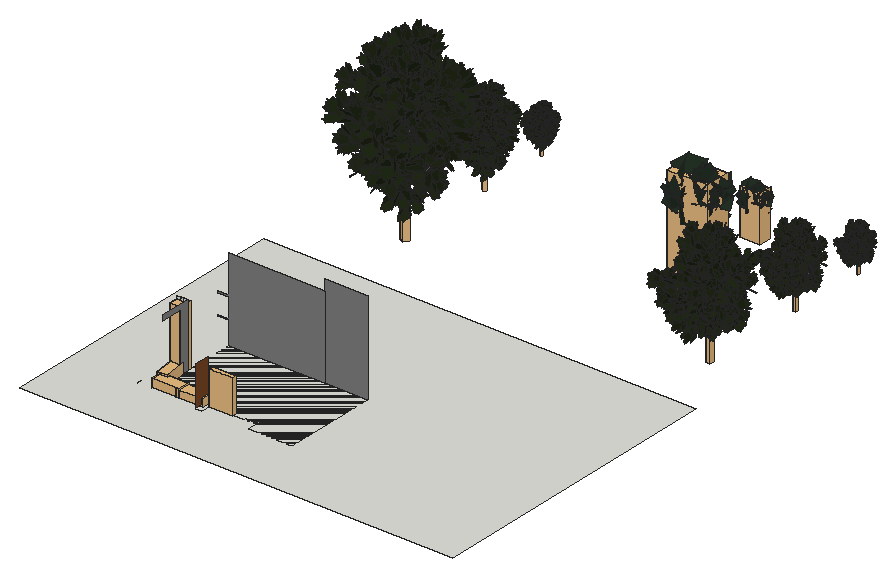
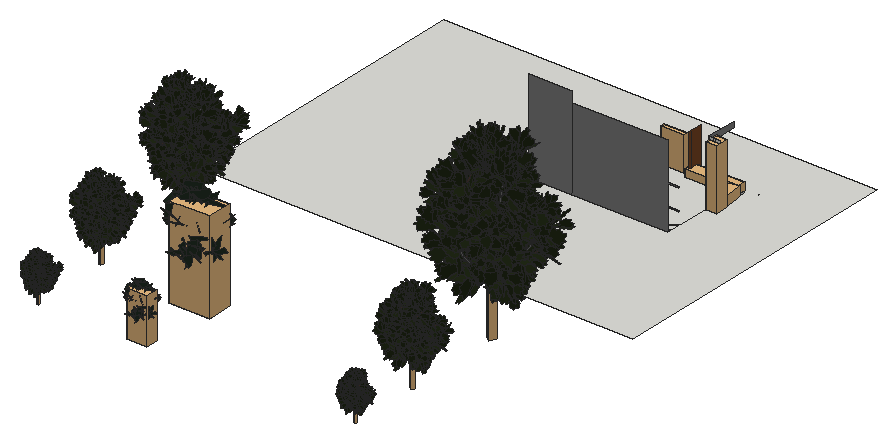
# SketchUp Ruby script. Lengths in inches.
U = 1.inch
M = Sketchup.active_model
def pt(a) = Geom::Point3d.new(a.map { |v| v * U })
def face(e, loops, mat)
  f = e.add_face(loops[0].map { |a| pt(a) })
  loops[1..].each { |l| e.add_face(l.map { |a| pt(a) }).erase! }
  f.material = f.back_material = mat if mat
  f
end
# faces: each face lists its corners as indices into pts; further lists are holes
def faces(e, pts, list, mat = nil) = list.each { |f| face(e, (f[0].is_a?(Array) ? f : [f]).map { |l| l.map { |i| pts[i] } }, mat) }
# xy, xz, yz: faces in a plane at the given z, y or x. An outline is a flat list of corners, or four numbers for a rectangle; further outlines are holes
def ring(l) = l.size == 4 ? [[l[0], l[1]], [l[2], l[1]], [l[2], l[3]], [l[0], l[3]]] : l.each_slice(2).to_a
def flat(e, list, mat, &to3) = list.each { |f| face(e, (f[0].is_a?(Array) ? f : [f]).map { |l| ring(l).map { |u, v| to3.(u, v) } }, mat) }
def xy(e, z, list, mat = nil) = flat(e, list, mat) { |x, y| [x, y, z] }
def xz(e, y, list, mat = nil) = flat(e, list, mat) { |x, z| [x, y, z] }
def yz(e, x, list, mat = nil) = flat(e, list, mat) { |y, z| [x, y, z] }
def lines(e, pts, list) = list.each { |a, b| e.add_line(pt(pts[a]), pt(pts[b])) }
# prism: a flat outline (further loops are holes) pulled along v
def prism(e, loops, v, mat = nil)
  f = face(e, loops, mat); d = Geom::Vector3d.new(v.map { |x| x * U })
  f.pushpull(f.normal.samedirection?(d) ? d.length : -d.length)
end
def box(e, o, s, mat = nil) = prism(e, [[o, [o[0] + s[0], o[1], o[2]], [o[0] + s[0], o[1] + s[1], o[2]], [o[0], o[1] + s[1], o[2]]]], [0, 0, s[2]], mat)
def at(x, y, z, deg = 0) = Geom::Transformation.translation(pt([x, y, z])) * Geom::Transformation.rotation(ORIGIN, Z_AXIS, deg.degrees)
def axes(o, x, y, z) = Geom::Transformation.new([*x, 0, *y, 0, *z, 0, *pt(o).to_a, 1])
def part(name) = M.definitions.add(name)
# library, detail: a bought-in or finely detailed component or shape, given as its bounding box
def library(name, o, s) = part(name).tap { |d| box(d.entities, o, s) }
def detail(e, o, s) = box(e.add_group.entities, o, s)
def put(e, d, t, mat = nil) = e.add_instance(d, t).tap { |i| i.material = mat if mat }
def group(e, t, mat = nil) = e.add_group.tap { |g| g.transformation = t; g.material = mat if mat }.entities
root = M.entities
M.materials.add("Color_D09").color = [86, 59, 49]
M.materials.add("Door").color = [117, 63, 33]
M.materials.add("Green ash – green texture").color = [33, 41, 22]
M.materials.add("[0133_Gray]").color = [128, 128, 128]
M.materials.add("[Color_005]1").color = [114, 114, 114]
M.materials.add("[Grass Dark Green]").color = [106, 157, 55]
M.materials.add("[Wood Veneer 01]").color = [120, 70, 37]
M.materials.add("euc leaf02").color = [35, 48, 36]
c1 = part("Component\#32")
xz(c1.entities,0,[[2.54,0,9.87,0.64,10.99,2.07,11.4,3.42,15.13,2.28,14.48,4.31,16.14,5.21,16.14,6.08,19.81,7.28,19.6,9.67,17.45,11.49,17.45,12.16,18.82,14.37,17.48,14.37,14.41,13.66,14.41,15.23,12.5625,17.49,9.84,15.21,8.9,13.85,7.74,13.625,7.35,12.68,6.87,13.02,6.35,12.27,5.92,10.47,4.2,7.42,2.84,6.89,0,2.38,0.07,1.59,2.8125,4.94,3.37,3.59,2.54,3.37,2.12,2.22]],"Green ash – green texture")
c2 = part("Component\#31")
xz(c2.entities,0,[[1.1,0,1.61,0,2.73,1.11,4.34,2.72,5.21,6.36,5.85,7.16,6.35,6.9375,6.85,8.05,8.03,8.05,8.625,9.25,10.11,11.7,9.56,13.83,9.56,15.84,7.83,15.84,6.03,14.37,5.31,16.54,4.4375,17.39,1.45,14.31,0,9.15,1.4,5.18,3.01,6.08,1.98,1.39]],"Green ash – green texture")
c3 = part("Component\#30")
put(c3.entities,c1,axes([0,7.77,0],[1,0,0],[0,0.89571,0.44464],[0,-0.44464,0.89571]))
put(c3.entities,c2,axes([2.15,6.37,5.26],[0.57629,-0.80824,0.12095],[0.79263,0.51673,-0.3236],[0.19905,0.28236,0.93843]))
c4 = part("Component\#33")
put(c4.entities,c3,axes([-4.97,-3.22,4.05],[0.69883,-0.69034,0.18725],[0.53248,0.3273,-0.7806],[0.47759,0.64522,0.59632]))
c5 = part("Component\#35")
put(c5.entities,c4,axes([0,5.2,2.2],[1,0,0],[0,0.90259,0.43051],[0,-0.43051,0.90259]))
c6 = part("leaf group 2")
put(c6.entities,c5,axes([-11.99,4.41,-4.35],[2.22014,-0.82385,1.14017],[1.36501,1.77637,-1.37441],[-0.33979,1.75315,1.92841]))
c7 = part("Component\#37")
put(c7.entities,c6,axes([-5.27,11.65,1.68],[-0.48323,0.10636,-0.43072],[-0.11515,-0.64511,-0.03012],[-0.42845,0.05342,0.49388]))
c8 = part("Component\#36")
xz(c8.entities,0,[[0.64,0,0,0.1875,4.21,2.81,8.59,4.11,12.8,4.11,19.57,2.81,12.8,3.73,8.59,3.73,4.21,2.3125]],"Color_D09")
c9 = part("Leafy twig")
put(c9.entities,c7,axes([23.53,12.57,24.85],[0.06536,-0.90475,-0.42089],[0.61791,-0.2945,0.72901],[-0.78353,-0.30772,0.53981]))
put(c9.entities,c7,axes([22.7,12.25,24.83],[-0.47146,-0.89493,0.11311],[0.80135,-0.48549,-0.35888],[0.36776,-0.0521,0.90651]))
put(c9.entities,c7,axes([24.25,0.65,20.83],[0.8253,-0.50372,0.24924],[0.23848,0.71461,0.65749],[-0.51157,-0.48438,0.71194]))
put(c9.entities,c7,axes([23.54,-2.45,18.63],[0.04689,-0.92492,0.3511],[0.72122,-0.28285,-0.64421],[0.71641,0.2674,0.65188]))
put(c9.entities,c7,axes([22.39,16.15,27.04],[-0.5311,-0.82173,0.2419],[0.41574,0.01583,0.89559],[-0.77461,0.50499,0.40813]))
put(c9.entities,c8,axes([22.76,-5.09,13.48],[0,1.66539,0.44624],[-1.72414,0,0],[0,-0.44624,1.66539]))
c10 = part("Bare twig")
p = [[0,0,0.13],[0.41,0.77,0],[4.07,2.79,10.125],[3.73,2.15,10.23],[7.66,4.77,23.875],[7.4,4.27,23.96],
  [8.6875,5.26,35.99],[8.5,4.91,36.05],[8.32,4.9375,46.95],[8.21,4.74,46.98]]
faces(c10.entities,p,[[0,1,2,3],[3,2,4,5],[4,6,7,5],[6,8,9,7]],"[Color_005]1")
c11 = part("Leafy twig \#1")
put(c11.entities,c10,axes([3.13,0.17,-0.45],[3.38032,6.88592,0.52481],[-5.85488,3.97559,0.303],[0,-1.35912,3.54524]))
put(c11.entities,c7,axes([0.37,31.375,148.94],[0.47772,0.64064,-1.51139],[2.85768,-0.62659,0.20284],[-0.43926,-3.3797,-0.3241]))
c12 = part("Ash branch")
put(c12.entities,c9,axes([28.11,72.66,46.26],[0.77413,-0.41274,-0.47998],[0.6311,0.56229,0.53435],[0.04934,-0.71657,0.69577]))
put(c12.entities,c9,axes([31.25,3.94,9.17],[0.73236,0.67893,0.05208],[-0.46223,0.55185,-0.69413],[-0.5,0.48428,0.71797]))
put(c12.entities,c9,axes([20.16,84.84,57.95],[0.96628,0.19619,0.16678],[-0.2575,0.73909,0.62245],[-0.00115,-0.6444,0.76469]))
put(c12.entities,c9,axes([30.13,29.18,11.93],[0.86603,0.2796,0.41452],[0,0.82904,-0.55919],[-0.5,0.48428,0.71797]))
put(c12.entities,c9,axes([47.67,28.63,-3.7],[0.1205,-0.71255,0.69119],[0.96646,0.24327,0.08231],[-0.2268,0.65809,0.71797]))
put(c12.entities,c9,axes([48.76,50.64,76.31],[-0.6716,0.46861,-0.57389],[0.01402,0.78248,0.62252],[0.74078,0.41004,-0.53209]))
put(c12.entities,c11,axes([42.34,0,10.34],[0.39368,0,0],[0,0.22544,-0.24092],[0,0.54032,0.50562]))
put(c12.entities,c9,axes([64.51,80.82,101.08],[-0.99604,0.06562,-0.06004],[-0.0106,0.58266,0.81265],[0.08831,0.81006,-0.57966]))
c13 = part("Ash branch \#2")
put(c13.entities,c9,axes([-3.64,36.17,23.18],[0.95801,0.10249,0.26779],[-0.28581,0.41631,0.86313],[-0.02302,-0.90343,0.42812]))
put(c13.entities,c9,axes([13.16,55.79,39.92],[0.70711,-0.61725,0.34497],[0,0.48786,0.87292],[-0.70711,-0.61725,0.34497]))
put(c13.entities,c11,axes([18.8125,5.17,0.46],[0.25503,0,0],[0,0.20007,-0.0752],[0,0.16866,0.44872]))
put(c13.entities,c9,axes([23.62,-10.17,21.5],[-0.56253,0.81775,0.12181],[0.38738,0.13053,0.91263],[0.73041,0.56057,-0.39021]))
put(c13.entities,c9,axes([45.18,27.18,68.96],[-0.96593,-0.22593,0.12627],[0.12295,0.02876,0.992],[-0.22775,0.97372,0]))
c14 = library("Tree trunk",[-6.35,9.4375,-76.57],[12.56,13.68,315.77])
c15 = part("Ash branch \#3")
put(c15.entities,c11,axes([21.47,3.93,0.22],[0.25503,0,0],[0,0.21068,-0.03601],[0,0.08077,0.47252]))
put(c15.entities,c9,axes([-4.05,13.6875,55.34],[0.70711,0.70373,-0.069],[0,0.09758,0.99523],[0.70711,-0.70373,0.069]))
put(c15.entities,c9,axes([6.52,33.54,18.07],[0.92587,-0.37604,0.03687],[0,0.09758,0.99523],[-0.37784,-0.92145,0.09035]))
c16 = part("Ash branch \#1")
put(c16.entities,c9,axes([26.17,74.02,40.56],[0.25882,-0.64004,0.72344],[0,0.74896,0.66262],[-0.96593,-0.1715,0.19384]))
put(c16.entities,c9,axes([6.38,24.03,55.81],[-0.04786,0.8645,-0.50035],[0.15558,0.50126,0.85119],[0.98666,-0.03711,-0.15849]))
put(c16.entities,c11,axes([17.68,0,1.01],[0.32282,0,0],[0,0.21407,-0.16545],[0,0.37107,0.48011]))
put(c16.entities,c9,axes([-9.1875,31.15,28.07],[0.82314,0.37626,-0.42529],[0,0.74896,0.66262],[0.56784,-0.54543,0.61649]))
put(c16.entities,c9,axes([0.54,-12.07,9.94],[0.19622,0.90478,-0.37799],[-0.67396,0.40444,0.61823],[0.71224,0.13344,0.68914]))
put(c16.entities,c9,axes([7.34,9.15,39.57],[0.05153,0.73872,-0.67204],[0.38679,0.60565,0.6954],[0.92072,-0.29578,-0.25452]))
put(c16.entities,c9,axes([36.2,51.23,15.73],[-0.18626,-0.35374,0.91661],[-0.31641,0.90483,0.2849],[-0.93016,-0.23696,-0.28046]))
c17 = part("Tree")
put(c17.entities,c12,axes([209.16,146.26,190.79],[-0.28773,1.46382,-0.87256],[-1.6259,0,0.48096],[0.49836,0.84514,1.51132]))
put(c17.entities,c12,axes([134.38,215.25,141.01],[1.59145,0,0],[0,1.58386,0.23671],[0,-0.32836,1.69393]))
put(c17.entities,c13,axes([178.04,237.71,388.46],[0,-1.63474,0],[1.63474,0,0],[0,0,1.78187]))
put(c17.entities,c12,axes([256.65,171.18,211.31],[-1.36815,1.04036,0],[-1.04036,-1.36815,0],[0,0,1.87346]))
put(c17.entities,c12,axes([167.11,160.33,284.63],[0.63716,1.20925,-0.47341],[-1.25908,0.71729,0.13762],[0.43501,0.34501,1.46674]))
put(c17.entities,c14,axes([199.97,188.06,127.43],[1.59145,0,0],[0,1.59145,0],[0,0,1.66425]))
put(c17.entities,c12,axes([275.77,218.4,281.93],[-1.57517,-0.28132,-0.44593],[0.06295,-1.50318,0.62621],[-0.42383,0.67416,1.53786]))
put(c17.entities,c12,axes([190.14,288,146.64],[0.35111,-1.78964,0],[1.72866,0.33915,0.47202],[-0.50488,-0.09905,1.92016]))
put(c17.entities,c12,axes([257.54,236.65,165.53],[-1.29152,-0.54158,0],[0.54158,-1.29152,0],[0,0,1.52652]))
put(c17.entities,c12,axes([175.36,274.13,265.04],[0.47642,-1.31213,-0.12271],[1.30597,0.45529,0.24003],[-0.16973,-0.17989,1.50253]))
put(c17.entities,c13,axes([228.65,212.14,385.35],[-1.53723,0.39369,-0.12111],[-0.39786,-1.55122,0.00748],[-0.10661,0.11241,1.71849]))
put(c17.entities,c15,axes([179.375,247.82,455.73],[0.79573,-1.37824,0],[1.37824,0.79573,0],[0,0,1.73468]))
put(c17.entities,c15,axes([220.2,190.4,436.52],[-0.90108,1.29724,0.19482],[-1.26794,-0.9219,0.27414],[0.36658,0,1.69551]))
put(c17.entities,c16,axes([195.4,185.625,330.61],[0,1.80471,0],[-1.731,0,0.5105],[0.55644,0,1.88679]))
put(c17.entities,c16,axes([180.07,237.23,322.66],[1.03006,-1.73903,-0.39964],[1.71651,0.8636,0.79163],[-0.4607,-0.67055,2.05597]))
put(c17.entities,c12,axes([252.86,167.09,121.2],[-1.29065,1.04142,0.30989],[-1.03312,-1.28343,0.15838],[0.47872,-0.11505,1.68865]))
put(c17.entities,c12,axes([145.45,238.15,252.03],[1.32497,-0.45364,0],[0.45364,1.32497,0],[0,0,1.52652]))
put(c17.entities,c16,axes([222.54,228.83,294],[-1.20488,-1.04179,0.83261],[1.23186,-1.24114,0.27288],[0.38905,0.70343,1.7146]))
put(c17.entities,c16,axes([223.77,224.36,314.875],[-1.40575,-0.68986,-0.30962],[0.56266,-1.37824,0.6133],[-0.4899,0.39658,1.59284]))
put(c17.entities,c16,axes([166.75,216.1,346.53],[1.65511,0,0],[0,1.6365,0.2475],[0,-0.26977,1.78379]))
put(c17.entities,c13,axes([162.33,209.39,372.71],[1.56679,-0.27909,0],[0.27909,1.56679,0],[0,0,1.73468]))
put(c17.entities,c13,axes([203.35,171.86,386.35],[0.15996,1.63137,0],[-1.63137,0.15996,0],[0,0,1.78672]))
c18 = part("Green Ash")
put(c18.entities,c14,axes([99.99,94.03,63.71],[0.79573,0,0],[0,0.79573,0],[0,0,0.83213]))
put(c18.entities,c13,axes([101.67,85.93,193.17],[0.07998,0.81569,0],[-0.81569,0.07998,0],[0,0,0.89336]))
put(c18.entities,c13,axes([89.02,118.86,194.23],[0,-0.81737,0],[0.81737,0,0],[0,0,0.89093]))
put(c18.entities,c12,axes([137.88,109.2,140.96],[-0.78759,-0.14066,-0.22296],[0.03147,-0.75159,0.31311],[-0.21191,0.33708,0.76893]))
put(c18.entities,c12,axes([67.1875,107.625,70.5],[0.79573,0,0],[0,0.79193,0.11835],[0,-0.16418,0.84696]))
put(c18.entities,c12,axes([104.58,73.13,95.39],[-0.14386,0.73191,-0.43628],[-0.81295,0,0.24048],[0.24918,0.42257,0.75566]))
put(c18.entities,c12,axes([128.33,85.59,105.66],[-0.68407,0.52018,0],[-0.52018,-0.68407,0],[0,0,0.93673]))
put(c18.entities,c12,axes([128.77,118.32,82.77],[-0.64576,-0.27079,0],[0.27079,-0.64576,0],[0,0,0.76326]))
put(c18.entities,c13,axes([114.32,106.07,192.67],[-0.76861,0.19684,-0.06056],[-0.19893,-0.77561,0.00374],[-0.0533,0.05621,0.85925]))
put(c18.entities,c12,axes([83.56,80.16,142.32],[0.31858,0.60462,-0.23671],[-0.62954,0.35865,0.06881],[0.21751,0.1725,0.73337]))
put(c18.entities,c13,axes([81.16,104.7,186.36],[0.7834,-0.13954,0],[0.13954,0.7834,0],[0,0,0.86734]))
put(c18.entities,c16,axes([97.7,92.8125,165.31],[0,0.90235,0],[-0.8655,0,0.25525],[0.27822,0,0.94339]))
put(c18.entities,c12,axes([87.68,137.07,132.52],[0.23821,-0.65607,-0.06135],[0.65299,0.22764,0.12002],[-0.08486,-0.08995,0.75126]))
put(c18.entities,c15,axes([89.6875,123.91,227.86],[0.39786,-0.68912,0],[0.68912,0.39786,0],[0,0,0.86734]))
put(c18.entities,c12,axes([95.07,144,73.32],[0.17556,-0.89482,0],[0.86433,0.16957,0.23601],[-0.25244,-0.04953,0.96008]))
put(c18.entities,c15,axes([110.1,95.2,218.26],[-0.45054,0.64862,0.09741],[-0.63397,-0.46095,0.13707],[0.18329,0,0.84775]))
put(c18.entities,c16,axes([90.03,118.62,161.33],[0.51503,-0.86951,-0.19982],[0.85825,0.4318,0.39581],[-0.23035,-0.33528,1.02798]))
put(c18.entities,c16,axes([83.38,108.05,173.27],[0.82756,0,0],[0,0.81825,0.12375],[0,-0.13489,0.89189]))
put(c18.entities,c16,axes([111.27,114.42,147],[-0.60244,-0.5209,0.41631],[0.61593,-0.62057,0.13644],[0.19452,0.35171,0.8573]))
put(c18.entities,c12,axes([126.43,83.55,60.6],[-0.64533,0.52071,0.15494],[-0.51656,-0.64172,0.07919],[0.23936,-0.05752,0.84432]))
put(c18.entities,c16,axes([111.89,112.18,157.4375],[-0.70287,-0.34493,-0.15481],[0.28133,-0.68912,0.30665],[-0.24495,0.19829,0.79642]))
put(c18.entities,c12,axes([72.73,119.08,126.01],[0.66249,-0.22682,0],[0.22682,0.66249,0],[0,0,0.76326]))
c19 = library("Group8",[-183.25,9.15,0],[25.91,56.79,43.93])
c20 = library("Group13",[-203.48,36.63,0],[29.68,67.31,50.64])
c21 = part("House+plant_11")
xy(c21.entities,0,[[-51.0625,-134.25,1040.6875,632.93]])
put(c21.entities,c19,at(-20.85,102.1,-20.91,-173.7))
put(c21.entities,c20,at(112.35,-141.89,-30.93,-90))
put(c21.entities,c20,at(172.12,-141.81,-32.82,-90))
c22 = library("GoldenBamboo",[-21.19,-21.7,-0.46],[44.22,41.02,72.81])
c23 = library("Group\#3",[0,0,0],[259.75,161.77,589.29])
c24 = part("Blue Gum")
p = [[271.53,158.18,378.25],[270.5625,158.71,380.69],[270.37,158.83,381.17],[272.73,162.06,384.51],[213.85,150.08,152.75],[212.24,149.06,149.65],
  [150.49,110.24,344.32],[151.97,108.18,342.21],[217.47,152.58,206.91],[209.32,150.04,213.6],[153.27,112.37,338.72],[213.34,156.04,223.13],
  [212.17,155.27,219.89],[213.66,148.52,337.14],[212.6875,151.94,345.88],[201.33,160.36,0],[198.82,151.26,0.01],[228.58,150.59,468.55],
  [228.91,150.53,474.28],[226.95,148.99,472.86]]
faces(c24.entities,p,[[0,1,2],[1,0,3],[3,2,1]])
lines(c24.entities,p,[[4,5],[6,7],[8,9],[10,6],[7,10],[11,12],[13,14],[15,16],[17,18],[19,17],[18,19]])
put(c24.entities,c23,axes([324.42,234.92,0.08],[-1,0,-0.00067],[0,-1,0.00003],[-0.00067,0.00003,1]))
g1 = group(c24.entities,at(392.72,299.04,214.24))
p = [[-190.24,-45.24,49.75],[-155.8,-83.51,-0.1],[-171.1,-117.4,15.86],[-186.4,-151.3,31.82],[-220.85,-113.03,81.67],[-197.84,-62.08,57.68],
  [-156.97,-85.38,90],[-134.58,-101.98,23.98],[-207.62,-132.83,7.74],[-230.01,-116.24,73.77],[-175.11,-93.05,85.97],[-155.875,-47.35,89.82],
  [-171.875,-81.0625,28.63],[-175.09,-115.85,49.06],[-178.3125,-150.63,69.48],[-162.3125,-116.92,130.67],[-157.47,-64.63,99.96],[-108.86,-93.44,91.87],
  [-142.19,-103.1875,29.18],[-207.99,-128.51,68.93],[-174.66,-118.76,131.62],[-125.2,-99.73,101.74],[-105.25,-143.93,101.02],[-118.65,-122.91,33.83],
  [-139.46,-91.34,48.24],[-160.28,-59.76,62.65],[-146.87,-80.78,129.84],[-115.59,-128.24,108.18],[-69.65,-64.39,98.91],[-102.98,-74.13,36.22],
  [-135.88,-86.79,56.09],[-168.78,-99.45,75.97],[-135.45,-89.7,138.66],[-85.99,-70.68,108.78],[-206,0,112.1],[-205.51,-55.1,41.09],
  [-219.69,-93.37,71.26],[-233.87,-131.63,101.43],[-234.36,-76.53,172.4375],[-220.18,-38.26,142.27],[-213.05,-19.01,127.09],[-58.99,-92.56,99.73],
  [-109.77,-114.37,54.1],[-132.54,-82.69,64.86],[-155.3,-51.01,75.61],[-104.53,-29.2,121.24],[-70.31,-76.82,105.07],[-84.85,-14.67,104.44],
  [-93.72,-70.0625,59.84],[-130.5,-76.32,75.5],[-167.29,-82.57,91.16],[-158.42,-27.18,135.76],[-103.12,-17.78,112.22],[-170.99,-48.24,149.78],
  [-170.5,-103.34,78.77],[-268.88,-83.39,63.75],[-269.37,-28.29,134.76],[-195.43,-43.28,146.05],[-119.44,-162.62,158.17],[-165.08,-157.98,109.24],
  [-139.69,-139.86,87.75],[-114.31,-121.74,66.26],[-68.68,-126.38,115.19],[-94.0625,-144.5,136.68],[-106.83,-153.62,147.5],[-83.43,-178.22,123.11],
  [-129.0625,-173.58,74.18],[-150.32,-106.13,101.32],[-104.69,-110.78,150.25],[-88.71,-161.47,129.85],[-153.18,-33.52,154.23],[-187.55,-61.6,76.08],
  [-205.14,-103.18,99.27],[-222.72,-144.75,122.47],[-188.35,-116.67,200.62],[-170.77,-75.09,177.42],[-161.92,-54.17,165.75],[-126.95,-97.9375,165.85],
  [-161.32,-126.02,87.7],[-248.95,-80.33,110.85],[-214.58,-52.25,189],[-148.72,-86.59,171.6],[-365.27,-93.53,149.96],[-339.43,-156.16,87.91],
  [-290.4375,-139.67,92.34],[-241.45,-123.17,96.77],[-267.29,-60.54,158.83],[-340.93,-85.33,152.16],[-220,-209.94,88.83],[-192.18,-284.625,134.55],
  [-202.3,-275.33,156.35],[-232.93,-247.2,222.33],[-260.75,-172.52,176.61],[-240.375,-191.23,132.72],[-392.72,-100.24,198.19],[-366.88,-162.88,136.14],
  [-328.26,-131.57,121.3],[-289.64,-100.27,106.47],[-315.48,-37.63,168.52],[-373.54,-84.69,190.82],[-327.95,-161.62,221.67],[-317.1,-180.89,132.49],
  [-328.31,-131.57,120.9375],[-339.53,-82.25,109.39],[-350.38,-62.97,198.5625],[-333.52,-137.11,215.93],[-255.83,-236.76,152.47],[-329.61,-198.39,191.52],
  [-323.5,-175.58,181.2],[-305,-106.55,149.96],[-231.21,-144.93,110.9],[-243.52,-190.85,131.6875],[-205.5,-81.8,220.89],[-197.86,-85.86,131.43],
  [-243.5,-64.11,127],[-289.13,-42.35,122.57],[-296.77,-38.29,212.03],[-251.13,-60.04,216.46],[-228.17,-70.99,218.6875],[-234.33,-241.65,142.48],
  [-225.25,-222.09,231.79],[-228.94,-197.05,226.92],[-240.1,-121.29,212.17],[-249.18,-140.85,122.86],[-241.75,-191.25,132.67],[-227.68,-15.04,215.96],
  [-220.04,-19.1,126.5],[-266.95,-109.11,127.5],[-274.59,-105.04,216.95],[-239.33,-37.4,216.21],[-312.18,-35.14,201.88],[-307.82,-106.7,144.42],
  [-256.66,-99.36,139.9],[-205.5,-92.02,135.375],[-209.86,-20.46,192.83],[-286.77,-31.49,199.63],[-224.25,-107.3,143.78],[-158.47,-57.42,184.1],
  [-153.89,-76.52,200.79],[-140.05,-134.32,251.29],[-205.83,-184.2,210.96],[-215.04,-145.75,177.37],[-371.18,-63.42,218.95],[-318.87,-74.08,144.18],
  [-278.67,-86.3125,174.61],[-238.47,-98.55,205.04],[-290.78,-87.88,279.82],[-351.21,-69.49,234.07],[-314.82,-59.28,247.3],[-323.0625,-96.32,163.62],
  [-272.16,-89.61,156.15],[-221.26,-82.9,148.67],[-213.02,-45.87,232.35],[-289.54,-55.95,243.59],[-269.6,-260.65,169.64],[-261.02,-289.45,256.47],
  [-255.15,-265.53,264.0625],[-237.36,-193.15,287.04],[-245.94,-164.36,200.22],[-257.77,-212.5,184.93],[-219.98,-94.58,184.38],[-135.38,-92.14,220.14],
  [-132.93,-117.5625,216.66],[-125.5,-194.48,206.12],[-210.1,-196.92,170.36],[-242.72,-259.5,171.19],[-311.27,-292.91,222.44],[-317.8125,-269.04,229.65],
  [-337.62,-196.84,251.48],[-269.07,-163.43,200.23],[-255.89,-211.46,185.71],[-204.01,-188.2,177.79],[-188.33,-208.64,265.98],[-194.51,-184.59,272.89],
  [-213.23,-111.83,293.8125],[-228.92,-91.39,205.62],[-216.46,-139.79,191.7],[-111.12,-172.19,178.4],[-144.16,-223.61,247],[-146.96,-202.62,261.69],
  [-155.45,-139.1,306.14],[-122.41,-87.68,237.53],[-116.76,-129.9375,207.97],[-92.3,-219.25,321.53],[-140.07,-175.86,256.125],[-105.48,-191.84,220.91],
  [-70.89,-207.83,185.69],[-23.13,-251.22,251.1],[-75.12,-227.1875,304.03],[-95.32,-86.56,260.02],[-28.15,-67.53,258.27],[-24.95,-79.6,243.18],
  [-15.25,-116.11,197.51],[-82.42,-135.13,199.26],[-88.87,-110.84,229.64],[-230.35,-182.42,199.75],[-240.26,-200.67,289.25],[-235.09,-176.09,295.07],
  [-219.44,-101.74,312.67],[-209.53,-83.5,223.17],[-219.9375,-132.96,211.46],[-140.68,-151.65,266.01],[-78.24,-142.94,332.84],[-63.08,-129.17,317.2],
  [-17.2,-87.5,269.85],[-79.64,-96.22,203.02],[-110.16,-123.93,234.52],[-181.78,-155.46,254.29],[-197.87,-106.1875,330.15],[-215.8125,-92.48,317.72],
  [-270.1,-51.01,280.11],[-254.02,-100.28,204.25],[-217.9,-127.875,229.27],[-219.05,-237.83,228.68],[-246.19,-265.11,312.11],[-270.4375,-258.25,306.72],
  [-343.82,-237.49,290.4],[-316.68,-210.21,206.96],[-267.86,-224.02,217.82],[-221.64,-245.99,220.16],[-255.74,-296.14,289.1875],[-278.74,-284.87,286.3125],
  [-348.35,-250.78,277.61],[-314.25,-200.64,208.59],[-267.95,-223.32,214.37],[-214.08,-176.63,246.6],[-287.9,-162.75,299.5],[-289.8,-138.53,290.89],
  [-295.55,-65.24,264.85],[-221.72,-79.12,211.94],[-273.56,-277.41,225.52],[-332.72,-264.05,294.53],[-330.67,-238.52,291.65],[-324.47,-161.27,282.95],
  [-265.3,-174.62,213.93],[-269.43,-226.01,219.72],[-125.42,-280.5,273.74],[-154.49,-208.42,224.74],[-56.47,-175.26,217.08],[-27.39,-247.34,266.08],
  [-101.07,-272.26,271.84],[-137.08,-126.63,220.68],[-181.31,-63.4,270.55],[-159.07,-51.25,275.29],[-91.8,-14.51,289.63],[-47.57,-77.74,239.76],
  [-92.33,-102.1875,230.22],[-238.16,-243.49,222.62],[-218.34,-248.07,312.22],[-217.08,-222.36,313.49],[-213.28,-144.56,317.34],[-233.09,-139.97,227.74],
  [-235.625,-191.73,225.18],[-96.8,-128.7,236.99],[-25.62,-162.74,224.18],[-29.7,-177.8,240.28],[-42.05,-223.37,289.02],[-113.23,-189.33,301.82],
  [-105.01,-159.01,269.41],[-190.11,-164.1875,296.41],[-166.86,-101.93,340.84],[-154.3,-94.29,323.91],[-116.3,-71.16,272.67],[-139.55,-133.41,228.25],
  [-164.83,-148.8,262.33],[-190.89,-165.45,228.74],[-213.01,-227.55,273.96],[-199.51,-220.6,290.46],[-158.68,-199.56,340.39],[-136.56,-137.46,295.18],
  [-163.73,-151.45,261.96],[-108.84,-65.86,242.35],[-143.91,-74.96,326.78],[-145.22,-100.52,323.73],[-149.17,-177.86,314.51],[-114.09,-168.76,230.08],
  [-111.47,-117.3125,236.21],[-131.79,-76.12,256.875],[-89.01,-36.19,327.71],[-66.95,-47.86,321.26],[-0.2,-83.16,301.74],[-42.99,-123.09,230.91],
  [-87.39,-99.61,243.89],[-191.96,-179.86,282.46],[-135.02,-196.07,336.18],[-121.21,-181.46,326.24],[-79.42,-137.25,296.18],[-136.36,-121.05,242.47],
  [-164.16,-150.45,262.47],[-230.13,-253.21,246.97],[-260.13,-299.04,320.74],[-267.04,-276.89,331.97],[-287.96,-209.88,365.95],[-257.97,-164.06,292.17],
  [-244.05,-208.64,269.57],[-280.97,-237.22,246.96],[-334.39,-225.07,320.72],[-316.05,-210.87,331.95],[-260.54,-167.9,365.9375],[-207.12,-180.05,292.18],
  [-123.3,-254.01,336.04],[-125.12,-228.29,247.85],[-81.63,-201.01,255.39],[-38.14,-173.74,262.92],[-36.32,-199.46,351.11],[-101.69,-240.46,339.78],
  [-68.26,-134.5,260.14],[-26.24,-201.97,251.74],[-44.5,-214.15,256.34],[-99.74,-251,270.27],[-141.76,-183.53,278.67],[-121.3,-170.4,347.79],
  [-129.86,-181.96,257.04],[-33.4,-220.07,253.73],[-24.85,-208.51,344.48],[-97.34,-179.87,346.97],[-78.09,-121.04,341.08],[-129.1,-143.71,268.11],
  [-128.64,-193.18,283.74],[-128.18,-242.65,299.36],[-77.17,-219.98,372.34],[-77.86,-145.61,348.85],[-177.42,-71.46,329.51],[-152.53,-122.65,273.39],
  [-155.7,-156.33,303.27],[-158.88,-190.01,333.16],[-183.78,-138.82,389.27],[-179,-88.19,344.35],[-150.51,-90.39,274.04],[-160.0625,-83.41,365.16],
  [-137.04,-94.48,368.65],[-67.4,-127.95,379.21],[-57.85,-134.93,288.09],[-104.18,-112.66,281.07],[-94.02,-187.3,327.96],[-81.13,-138.55,389.98],
  [-69.09,-124.83,376.95],[-32.66,-83.33,337.53],[-45.54,-132.09,275.51],[-69.78,-159.69,301.74],[-118.35,-128.14,277.49],[-134.07,-116.2,367.22],
  [-118.18,-95.9,367.54],[-70.12,-34.49,368.49],[-54.4,-46.4375,278.76],[-86.375,-87.29,278.12],[-130.67,-185.64,278.8125],[-99.69,-223.89,341.79],
  [-81.85,-210.3,341.52],[-27.87,-169.2,340.6875],[-58.85,-130.95,277.71],[-94.76,-158.29,278.26],[-124.09,-168.51,302.87],[-98.25,-187.53,376.08],
  [-77.34,-181.72,370.43],[-14.08,-164.14,353.32],[-39.93,-145.12,280.11],[-82.01,-156.82,291.49],[-222.9,-199.13,376.1],[-220.07,-149.45,341.44],
  [-227.34,-168.57,313.98],[-234.62,-187.6875,286.52],[-237.45,-237.37,321.18],[-230.17,-218.25,348.64],[-226.51,-208.63,362.46],[-66.91,-203,314.13],
  [-2.98,-185.26,358.72],[-4.41,-163.74,352.56],[-8.73,-98.64,333.94],[-72.66,-116.39,289.35],[-169.41,-164.76,388.4],[-177.97,-176.3125,297.65],
  [-129.74,-195.37,296],[-81.52,-214.43,294.34],[-72.96,-202.87,385.09],[-145.46,-174.22,387.58],[-154.72,-129.21,384.88],[-129.15,-146.67,298.38],
  [-129.71,-197.46,308.96],[-130.27,-248.25,319.53],[-155.84,-230.78,406.04],[-155,-154.4375,390.14],[-202.43,-168.15,321.54],[-179.78,-204.63,388.96],
  [-158.3,-199.98,384.5],[-93.32,-185.9,371.01],[-115.96,-149.42,303.58],[-159.19,-158.79,312.5625],[-197.46,-225.01,341.1],[-194.63,-175.33,306.4375],
  [-260.05,-161.8125,321.53],[-262.88,-211.49,356.1875],[-213.71,-221.65,344.85],[-157.48,-194.21,341.46],[-113.86,-228.8,398.82],[-95.37,-218.73,391.1],
  [-39.42,-188.27,367.76],[-83.04,-153.67,310.41],[-120.26,-173.9375,325.9375],[-193.32,-187.43,311.78],[-211.98,-162.83,385.51],[-194.23,-149.13,385.64],
  [-140.53,-107.67,386.06],[-121.86,-132.27,312.33],[-157.59,-159.85,312.05],[-258.44,-158.87,437.95],[-244.84,-121.05,355.33],[-234.18,-168.04,336.09],
  [-223.52,-215.03,316.85],[-237.12,-252.84,399.47],[-253.15,-182.21,428.39],[-193.45,-225.28,404.25],[-172.56,-175.18,330.125],[-129.23,-203.0625,324.0625],
  [-85.9,-230.95,318],[-106.8,-281.05,392.12],[-171.93,-239.14,401.24],[-189.32,-183.99,368.07],[-165.25,-149.36,435.97],[-148.5625,-139.1,425.06],
  [-98.07,-108.05,392.03],[-122.15,-142.68,324.13],[-155.73,-163.33,346.1],[-155.65,-206.76,334.06],[-167.83,-218.04,412.25],[-167.96,-195.875,415.63],
  [-168.38,-128.8,425.86],[-156.21,-117.52,347.67],[-155.93,-162.14,340.86],[-145.4375,-206.81,336.52],[-133.41,-216.07,415],[-138.07,-194.41,418.47],
  [-152.15,-128.87,428.97],[-164.18,-119.61,350.49],[-154.81,-163.21,343.5],[-277.65,-112.64,443.48],[-209.06,-142.23,389.99],[-242.625,-172.43,364.44],
  [-276.2,-202.63,338.89],[-344.79,-173.04,392.38],[-294.33,-127.64,430.79],[-116.84,-180.91,416.6],[-166.69,-214.06,346.91],[-201.41,-176.24,354.36],
  [-236.13,-138.41,361.82],[-186.28,-105.26,431.51],[-134.09,-162.12,420.31],[-150.67,-209.23,358.7],[-156.56,-222.56,437.29],[-138.24,-210.16,440.97],
  [-82.8125,-172.64,452.1],[-76.93,-159.31,373.5],[-113.8,-184.27,366.1],[-154.14,-165.42,373.5],[-127.09,-136.44,442.91],[-107.04,-145.81,439.23],
  [-46.4,-174.14,428.11],[-73.46,-203.11,358.7],[-161.71,-108.91,440.68],[-158.5,-155.86,361.76],[-202.41,-180.14,374.96],[-246.32,-204.43,388.15],
  [-249.52,-157.48,467.07],[-183.52,-120.98,447.23]]
faces(g1,p,[[0,1,2,3,4,5],[6,7,2,8,9,10],[11,12,13,14,15,16],[17,18,13,19,20,21],[22,23,24,25,26,27],[28,29,30,31,32,33],[34,35,36,37,38,39,40],[41,42,43,44,45,46],
  [47,48,49,50,51,52],[53,54,36,55,56,39,57],[58,59,60,61,62,63,64],[65,66,60,67,68,63,69],[70,71,72,73,74,75,76],[77,78,72,79,80,75,81],[82,83,84,85,86,87],[88,89,90,91,92,93],
  [94,95,96,97,98,99],[100,101,102,103,104,105],[106,107,108,109,110,111],[112,113,114,115,116,117,118],[119,120,121,122,123,124],[125,126,114,127,128,117,129],[130,131,132,133,134,135],[136,137,138,139,140,141],
  [142,143,144,145,146,147],[148,149,150,151,152,153],[154,155,156,157,158,159],[160,161,162,163,164,141],[165,166,167,168,169,170],[171,172,173,174,175,176],[177,178,179,180,181,182],[183,184,185,186,187,188],
  [189,190,191,192,193,194],[195,196,197,198,199,200],[201,202,203,204,205,206],[207,208,209,210,211,212],[213,214,215,216,217,218],[219,220,221,222,223,224],[225,226,227,228,229,212],[230,231,232,233,234,235],
  [236,237,185,238,239,240],[241,242,243,244,245,246],[247,248,249,250,251,252],[253,254,255,256,257,258],[259,260,261,262,263,264],[265,266,267,268,269,270],[271,272,273,274,275,276],[277,278,279,280,281,282],
  [283,284,285,286,287,288],[289,290,291,292,293,294],[295,296,297,298,299,294],[300,301,302,303,304,305],[306,307,308,309,310,258],[311,312,302,313,314,315],[316,317,318,319,320,321],[322,323,324,325,326,327],
  [328,329,330,331,332,333],[334,335,336,337,338,339],[340,341,342,343,344,345],[346,347,348,349,350,351],[352,353,354,355,356,357],[358,359,360,361,362,363,364],[365,366,367,368,369,339],[370,371,372,373,374,375],
  [376,377,378,379,380,381],[382,383,384,385,386,387],[388,389,360,390,391,363,392],[393,394,395,396,397,398],[399,400,401,402,403,404],[405,406,407,408,409,410],[411,412,413,414,415,416],[417,418,419,420,421,422],
  [423,424,425,426,427,428],[429,430,431,432,433,434],[435,436,437,438,439,440],[441,442,443,444,445,446],[447,448,449,450,451,452],[453,454,455,456,457,452],[458,459,460,461,462,463]],"euc leaf02")
c25 = library("Door",[0,-42.93,0],[10.47,42.93,84.29])
xy(root,-3.125,[[553.86,173.38,679.09,173.38,679.09,183.7,564.49,183.7,564.49,261.08,553.86,261.08]],"[Grass Dark Green]")
xy(root,0,[[812.47,152.69,921.28,152.69,921.28,390.8,570.41,390.8,570.41,237.58,572.41,237.58,572.41,188.52,679.09,188.52,679.09,184.77,755.09,184.77,755.09,179.27,756.79,179.27,756.79,184.77,757.59,184.77,757.59,179.27,759.29,179.27,759.29,184.77,760.09,184.77,760.09,179.27,761.79,179.27,761.79,184.77,762.59,184.77,762.59,179.27,764.29,179.27,764.29,184.77,765.09,184.77,765.09,179.27,766.79,179.27,766.79,184.77,767.59,184.77,767.59,179.27,769.29,179.27,769.29,184.77,770.09,184.77,770.09,179.27,771.79,179.27,771.79,184.77,772.59,184.77,772.59,179.27,774.29,179.27,774.29,184.77,775.09,184.77,775.09,179.27,776.79,179.27,776.79,184.77,777.59,184.77,777.59,179.27,779.29,179.27,779.29,184.77,780.09,184.77,780.09,179.27,781.79,179.27,781.79,184.77,782.59,184.77,782.59,179.27,784.29,179.27,784.29,184.77,785.09,184.77,785.09,179.27,786.79,179.27,786.79,184.77,787.59,184.77,787.59,179.27,789.29,179.27,789.29,184.77,790.09,184.77,790.09,179.27,791.79,179.27,791.79,184.77,792.59,184.77,792.59,179.27,794.29,179.27,794.29,184.77,795.47,184.77,795.47,179.27,797.16,179.27,797.16,184.77,798.34,184.77,798.34,179.27,800.04,179.27,800.04,184.77,801.22,184.77,801.22,179.27,802.91,179.27,802.91,184.77,804.09,184.77,804.09,179.27,805.79,179.27,805.79,184.77,806.97,184.77,806.97,179.27,808.66,179.27,808.66,184.77,809.84,184.77,809.84,179.27,811.54,179.27,811.54,184.77,812.47,184.77],[679.09,152.69,694.73,184.77],[525.25,162.48,525.25,171.1,525.05,165.14],[564.49,183.7,564.74,248.89],[565.04,183.7,679.09,184.6],
  [565.41,237.58,570.41,241.02],[565.16,241.02,570.41,261.08],[542.91,261.08,570.41,273.58]])
xz(root,173.38,[[553.86,-3.125,679.09,1.5625]])
xz(root,179.27,[[809.84,0,811.54,1.5625]])
xz(root,183.7,[[564.49,-3.125,564.74,0],[564.74,-3.125,679.09,0],[565.04,0,679.09,9.25]])
xz(root,184.6,[[565.04,0,679.09,9.25]])
xz(root,184.77,[[808.66,0,809.84,1.5625],[811.54,0,812.47,1.5625]])
xz(root,237.58,[[565.04,0,565.41,9.25]])
xz(root,241.02,[[565.16,0,565.41,9.25],[565.41,0,570.41,146.5]])
xz(root,261.08,[[553.86,-3.125,554.03,0],[554.03,-3.125,555.09,0],[555.09,-3.125,564.49,0],[553.86,0,554.03,0,554.03,160.15,542.91,160.15,542.91,1.5625,553.86,1.5625],[554.03,0,555.09,160.15],
  [555.09,0,565.04,0,565.04,9.25,559.28,9.25,559.28,160.15,555.09,160.15],[565.16,0,570.41,0,570.41,160.15,560.36,160.15,560.36,9.25,565.16,9.25],[565.04,0,565.16,9.25]])
xz(root,390.8,[[570.41,0,570.41,56.77,542.91,56.77,542.91,59.17,570.41,59.17,570.41,110.22,542.91,110.22,542.91,113.5,570.41,113.5,570.41,208.1875,812.47,208.1875,812.47,0],[812.47,0,921.28,235.625]],"[0133_Gray]")
yz(root,553.86,[[173.38,-3.125,261.08,1.5625]])
yz(root,564.49,[[183.7,-3.125,248.89,0],[248.89,-3.125,261.08,0]])
yz(root,565.16,[[241.02,0,261.08,9.25]])
yz(root,565.41,[[237.58,0,241.02,9.25]])
yz(root,570.41,[[241.02,0,241.02,146.5,184.77,146.5,184.77,160.15,261.08,160.15,261.08,0]],"[0133_Gray]")
yz(root,679.09,[[173.38,-3.125,183.7,0],[183.7,0,184.6,9.25]])
yz(root,679.09,[[173.38,0,173.38,1.5625,152.69,1.5625,152.69,101.125,188.52,101.125,188.52,16.125,184.6,16.125,184.6,9.25,183.7,9.25,183.7,0]],"[Wood Veneer 01]")
yz(root,809.84,[[179.27,0,184.77,1.5625]])
yz(root,811.54,[[179.27,0,184.77,1.5625]])
p = [[677.34,185.64,101.125],[677.34,185.64,0],[572.41,184.77,0],[572.41,184.78,0]]
lines(root,p,[[0,1],[2,3]])
put(root,c17,axes([626.59,722.9375,0],[0.42475,0.62972,0],[-0.62972,0.42475,0],[0,0,0.75958]))
put(root,c18,at(1253.13,824.27,0))
put(root,c17,axes([598.95,1085.18,0],[0.21238,0.31486,0],[-0.31486,0.21238,0],[0,0,0.37979]))
put(root,c18,axes([1294.17,1121.89,2.93],[0.66,0,0],[0,0.66,0],[0,0,0.66]))
put(root,c18,axes([1321.14,1349.33,-0.07],[0.3828,0,0],[0,0.3828,0],[0,0,0.3828]))
put(root,c17,axes([587.49,1317.98,0],[0.10619,0.15743,0],[-0.15743,0.10619,0],[0,0,0.1899]))
put(root,c21,at(408.8,134.25,0))
put(root,c22,axes([555.8,256.52,0.51],[0.59,0,0],[0,0.79,0],[0,0,2.11]))
put(root,c24,axes([1034.78,1133.79,-0.06],[0.392,0,0],[0,0.392,0],[0,0,0.392]))
put(root,c24,axes([1071.63,1345.71,-0.08],[0.196,0,0],[0,0.196,0],[0,0,0.196]))
put(root,c25,axes([694.73,174.88,0],[0,1.02,0],[-1.3668,0,0],[0,0,1.02]))
